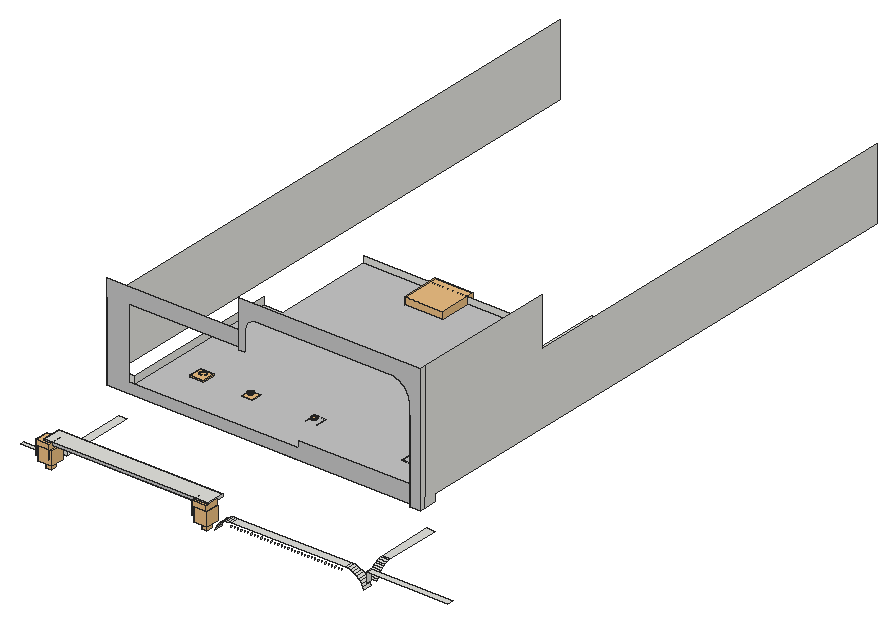
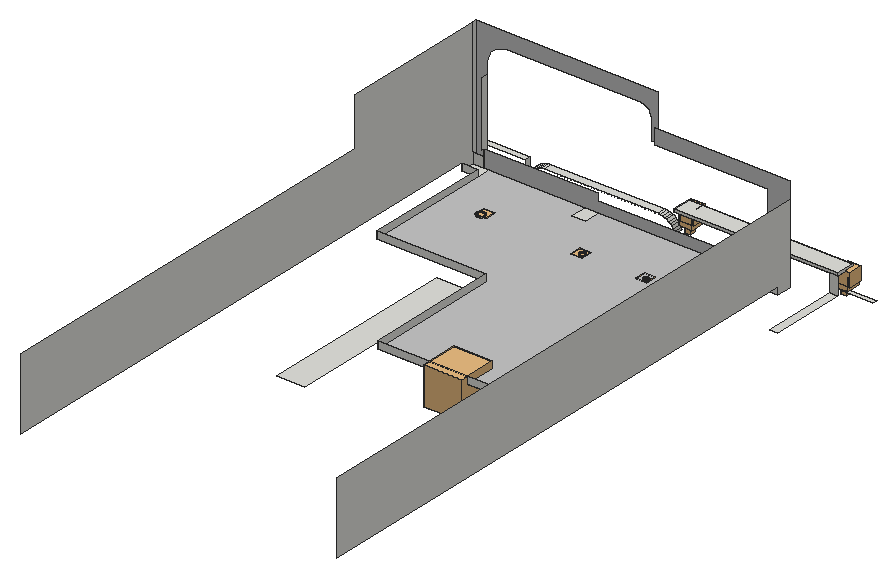
# SketchUp Ruby script. Lengths in inches.
U = 1.inch
M = Sketchup.active_model
def pt(a) = Geom::Point3d.new(a.map { |v| v * U })
def face(e, loops, mat)
  f = e.add_face(loops[0].map { |a| pt(a) })
  loops[1..].each { |l| e.add_face(l.map { |a| pt(a) }).erase! }
  f.material = f.back_material = mat if mat
  f
end
# faces: each face lists its corners as indices into pts; further lists are holes
def faces(e, pts, list, mat = nil) = list.each { |f| face(e, (f[0].is_a?(Array) ? f : [f]).map { |l| l.map { |i| pts[i] } }, mat) }
# xy, xz, yz: faces in a plane at the given z, y or x. An outline is a flat list of corners, or four numbers for a rectangle; further outlines are holes
def ring(l) = l.size == 4 ? [[l[0], l[1]], [l[2], l[1]], [l[2], l[3]], [l[0], l[3]]] : l.each_slice(2).to_a
def flat(e, list, mat, &to3) = list.each { |f| face(e, (f[0].is_a?(Array) ? f : [f]).map { |l| ring(l).map { |u, v| to3.(u, v) } }, mat) }
def xy(e, z, list, mat = nil) = flat(e, list, mat) { |x, y| [x, y, z] }
def xz(e, y, list, mat = nil) = flat(e, list, mat) { |x, z| [x, y, z] }
def yz(e, x, list, mat = nil) = flat(e, list, mat) { |y, z| [x, y, z] }
def lines(e, pts, list) = list.each { |a, b| e.add_line(pt(pts[a]), pt(pts[b])) }
# prism: a flat outline (further loops are holes) pulled along v
def prism(e, loops, v, mat = nil)
  f = face(e, loops, mat); d = Geom::Vector3d.new(v.map { |x| x * U })
  f.pushpull(f.normal.samedirection?(d) ? d.length : -d.length)
end
def box(e, o, s, mat = nil) = prism(e, [[o, [o[0] + s[0], o[1], o[2]], [o[0] + s[0], o[1] + s[1], o[2]], [o[0], o[1] + s[1], o[2]]]], [0, 0, s[2]], mat)
def at(x, y, z, deg = 0) = Geom::Transformation.translation(pt([x, y, z])) * Geom::Transformation.rotation(ORIGIN, Z_AXIS, deg.degrees)
def axes(o, x, y, z) = Geom::Transformation.new([*x, 0, *y, 0, *z, 0, *pt(o).to_a, 1])
def part(name) = M.definitions.add(name)
# library, detail: a bought-in or finely detailed component or shape, given as its bounding box
def library(name, o, s) = part(name).tap { |d| box(d.entities, o, s) }
def detail(e, o, s) = box(e.add_group.entities, o, s)
def put(e, d, t, mat = nil) = e.add_instance(d, t).tap { |i| i.material = mat if mat }
def group(e, t, mat = nil) = e.add_group.tap { |g| g.transformation = t; g.material = mat if mat }.entities
root = M.entities
M.materials.add("[Color M02]").color = [198, 198, 198]
M.materials.add("[Wood Floor Parquet]").color = [145, 89, 39]
c1 = library("Spot Light\#6",[-5.1,-5.1,-11.05],[10.2,10.2,11.05])
c2 = library("Omni Light\#11",[-12,-12,-12],[24,24,24])
c3 = library("Omni Light\#12",[-12,-12,-12],[24,24,24])
c4 = library("Omni Light\#13",[-12,-12,-12],[24,24,24])
c5 = library("Omni Light\#19",[-12,-12,-12],[24,24,24])
c6 = library("Omni Light\#18",[-12,-12,-12],[24,24,24])
c7 = library("Omni Light\#23",[-12,-12,-12],[24,24,24])
c8 = library("Omni Light\#20",[-12,-12,-12],[24,24,24])
c9 = library("Omni Light\#16",[-12,-12,-12],[24,24,24])
c10 = library("Omni Light\#17",[-12,-12,-12],[24,24,24])
c11 = library("Omni Light\#22",[-12,-12,-12],[24,24,24])
c12 = library("Omni Light\#15",[-12,-12,-12],[24,24,24])
c13 = library("Omni Light\#21",[-12,-12,-12],[24,24,24])
c14 = library("Omni Light\#14",[-12,-12,-12],[24,24,24])
c15 = library("Spot Light\#10",[-5.1,-5.1,-11.05],[10.2,10.2,11.05])
xy(root,48,[[52.9375,113,66.86,244.9375]])
xy(root,49.42,[[56.17,85.5625,62.99,89.5625],[330.61,85.5625,337.42,89.5625]],"[Color M02]")
xy(root,50.9375,[[0,94.125,52.9375,101.45]])
xy(root,61.1875,[[376.11,89.5625,576.66,104.0625],[596.33,146.41,610.25,244.9375]])
xy(root,61.98,[[56.17,85.5625,62.99,89.5625],[330.61,85.5625,337.42,89.5625]],"[Color M02]")
xy(root,63.75,[[610.25,94.125,754.3125,104.0625]])
xy(root,79.6875,[[52.9375,79.3125,66.86,89.5625],[66.86,79.3125,66.86,113,341.76,113,341.76,104.75,326.57,104.75,326.57,79.3125],[326.57,79.3125,341.76,89.5625],[52.9375,89.5625,66.86,113],[326.57,89.5625,341.76,104.75]])
xy(root,84,[[52.9375,79.3125,341.76,113],[427.3,467.53,475.3,820.03],[115.1,706.78,146.03,752.85],[181,706.78,229,752.85]])
xy(root,107.6875,[[591.56,213,610.25,219.25],[52.9375,219.25,80.78,244.9375],[388.4375,219.25,412.5,248.6],[582.4,219.25,610.25,244.9375]])
xy(root,107.6875,[[[80.78,219.25,80.78,529.39,115.1,529.39,115.1,706.78,388.8,706.78,388.8,467.53,582.4,467.53,582.4,219.25,412.5,219.25,412.5,248.6,388.4375,248.6,388.4375,219.25],[512.63,317.48,514.56,317.74,516.35,318.48,517.89,319.66,519.07,321.2,519.82,323,520.07,324.92,519.82,326.85,519.07,328.64,517.89,330.18,516.35,331.36,514.56,332.1,512.63,332.36,510.71,332.1,508.91,331.36,507.375,330.18,506.19,328.64,505.45,326.85,505.2,324.92,505.45,323,506.19,321.2,507.375,319.66,508.91,318.48,510.71,317.74],[333.76,319.66,335.12,319.84,336.39,320.37,337.48,321.2,338.3125,322.29,338.84,323.56,339.02,324.92,338.84,326.28,338.3125,327.55,337.48,328.64,336.39,329.47,335.12,330,333.76,330.18,332.4,330,331.13,329.47,330.04,328.64,329.21,327.55,328.68,326.28,328.5,324.92,328.68,323.56,329.21,322.29,330.04,321.2,331.13,320.37,332.4,319.84],[137.46,319.67,138.82,319.85,140.09,320.375,141.17,321.21,142.01,322.3,142.53,323.5625,142.71,324.92,142.53,326.28,142.01,327.55,141.17,328.63,140.09,329.47,138.82,329.99,137.46,330.17,136.1,329.99,134.84,329.47,133.75,328.63,132.91,327.55,132.39,326.28,132.21,324.92,132.39,323.5625,132.91,322.3,133.75,321.21,134.84,320.375,136.1,319.85],[221.33,320.11,222.57,320.27,223.73,320.75,224.73,321.52,225.5,322.51,225.98,323.67,226.14,324.92,225.98,326.17,225.5,327.33,224.73,328.32,223.73,329.09,222.57,329.57,221.33,329.73,220.08,329.57,218.92,329.09,217.92,328.32,217.16,327.33,216.68,326.17,216.51,324.92,216.68,323.67,217.16,322.51,217.92,321.52,218.92,320.75,220.08,320.27]]],"[Color M02]")
xz(root,79.3125,[[52.9375,79.6875,341.76,84]],"[Color M02]")
xz(root,85.5625,[[56.17,49.42,62.99,61.98],[330.61,49.42,337.42,61.98]],"[Wood Floor Parquet]")
xz(root,113,[[52.9375,48,66.86,79.6875],[52.9375,79.6875,341.76,84]])
xz(root,213,[[591.56,107.6875,610.25,107.6875,610.25,331.6875,290.41,331.6875,290.41,249.875,300.96,249.875,300.96,283.625,301.125,286.24,301.61,288.8125,302.41,291.31,303.52,293.68,304.91,295.9,306.5625,297.93,308.46,299.74,310.5625,301.3,312.84,302.58,315.27,303.58,317.79,304.26,320.39,304.625,554.68,304.625,559.5,304.31,564.23,303.37,568.79,301.82,573.12,299.6875,577.13,297.01,580.76,293.83,583.9375,290.2,586.62,286.19,588.75,281.87,590.3,277.3,591.24,272.57,591.56,267.76]],"[Color M02]")
xz(root,219.25,[[591.56,107.6875,610.25,126]])
xz(root,219.25,[[52.9375,107.6875,591.56,107.6875,591.56,138.5625,390.47,138.5625,390.47,126.375,91.81,126.375,91.81,246,91.94,246,91.94,249.875,290.41,249.875,290.41,277.0625,52.9375,277.0625]],"[Color M02]")
xz(root,244.9375,[[52.9375,107.6875,80.78,120],[582.4,107.6875,610.25,120]])
xz(root,467.53,[[388.8,107.6875,582.4,120]])
xz(root,706.78,[[115.1,107.6875,388.8,120]])
yz(root,52.9375,[[79.3125,79.6875,113,84],[219.25,107.6875,219.25,246,1217.1875,246,1217.1875,120,244.9375,120,244.9375,107.6875]])
yz(root,56.17,[[85.5625,49.42,89.5625,61.98]],"[Color M02]")
yz(root,62.99,[[85.5625,49.42,89.5625,61.98]],"[Wood Floor Parquet]")
yz(root,80.78,[[244.9375,107.6875,529.39,120]])
yz(root,330.61,[[85.5625,49.42,89.5625,61.98]],"[Color M02]")
yz(root,337.42,[[85.5625,49.42,89.5625,61.98]],"[Color M02]")
yz(root,341.76,[[79.3125,79.6875,113,84]])
yz(root,373.05,[[92.0625,52.27,92.8125,53.85]])
yz(root,378.96,[[92.0625,52.27,92.8125,54.05]])
yz(root,384.88,[[92.0625,52.27,92.8125,54.05]])
yz(root,388.8,[[467.53,107.6875,706.78,120]])
yz(root,390.79,[[92.0625,52.27,92.8125,54.05]])
yz(root,396.71,[[92.0625,52.27,92.8125,54.05]])
yz(root,402.625,[[92.0625,52.27,92.8125,54.05]])
yz(root,408.54,[[92.0625,52.27,92.8125,54.05]])
yz(root,414.45,[[92.0625,52.27,92.8125,54.05]])
yz(root,420.37,[[92.0625,52.27,92.8125,54.05]])
yz(root,426.28,[[92.0625,52.27,92.8125,54.05]])
yz(root,432.2,[[92.0625,52.27,92.8125,54.05]])
yz(root,438.11,[[92.0625,52.27,92.8125,54.05]])
yz(root,444.03,[[92.0625,52.27,92.8125,54.05]])
yz(root,449.94,[[92.0625,52.27,92.8125,54.05]])
yz(root,455.86,[[92.0625,52.27,92.8125,54.05]])
yz(root,461.77,[[92.0625,52.27,92.8125,54.05]])
yz(root,467.6875,[[92.0625,52.27,92.8125,54.05]])
yz(root,473.6,[[92.0625,52.27,92.8125,54.05]])
yz(root,479.52,[[92.0625,52.27,92.8125,54.05]])
yz(root,485.43,[[92.0625,52.27,92.8125,54.05]])
yz(root,491.35,[[92.0625,52.27,92.8125,54.05]])
yz(root,497.26,[[92.0625,52.27,92.8125,54.05]])
yz(root,503.18,[[92.0625,52.27,92.8125,54.05]])
yz(root,509.09,[[92.0625,52.27,92.8125,54.05]])
yz(root,515,[[92.0625,52.27,92.8125,54.05]])
yz(root,520.92,[[92.0625,52.27,92.8125,54.05]])
yz(root,526.83,[[92.0625,52.27,92.8125,54.05]])
yz(root,532.75,[[92.0625,52.27,92.8125,54.05]])
yz(root,538.66,[[92.0625,52.27,92.8125,54.05]])
yz(root,544.58,[[92.0625,52.27,92.8125,54.05]])
yz(root,550.49,[[92.0625,50.58,92.8125,52.27],[92.0625,52.27,92.8125,54.05]])
yz(root,556.41,[[92.0625,52.27,92.8125,54.05]])
yz(root,562.32,[[92.0625,52.27,92.8125,54.05]])
yz(root,568.24,[[92.0625,52.27,92.8125,54.05]])
yz(root,582.4,[[244.9375,107.6875,467.53,120]])
yz(root,591.56,[[213,107.6875,213,251.38,222.9375,251.38,222.9375,138.5625,219.25,138.5625,219.25,107.6875]])
yz(root,610.25,[[94.125,45.67,104.0625,63.75],[213,107.6875,219.25,107.6875,219.25,126,222.9375,126,222.9375,331.6875,213,331.6875],[219.25,107.6875,244.9375,107.6875,244.9375,120,1217.1875,120,1217.1875,246,479.76,246,479.76,331.6875,222.9375,331.6875,222.9375,126,219.25,126]])
p = [[607.69,104.0625,40.45],[607.69,89.5625,40.45],[609.11,89.5625,36.29],[609.11,104.0625,36.29],[346.56,104.0625,38.51],[346.56,89.5625,38.51],
  [347.85,89.5625,42.3],[347.85,104.0625,42.3],[610.25,116.85,38.51],[610.25,118.14,42.3],[596.33,118.14,42.3],[596.33,116.85,38.51],
  [605.75,104.0625,44.39],[605.75,89.5625,44.39],[349.62,89.5625,45.89],[349.62,104.0625,45.89],[610.25,119.91,45.89],[596.33,119.91,45.89],
  [603.31,104.0625,48.04],[603.31,89.5625,48.04],[351.84,89.5625,49.22],[351.84,104.0625,49.22],[610.25,122.13,49.22],[596.33,122.13,49.22],
  [600.41,104.0625,51.35],[600.41,89.5625,51.35],[354.48,89.5625,52.23],[354.48,104.0625,52.23],[610.25,124.77,52.23],[596.33,124.77,52.23],
  [597.11,104.0625,54.25],[597.11,89.5625,54.25],[357.49,89.5625,54.87],[357.49,104.0625,54.87],[610.25,127.78,54.87],[596.33,127.78,54.87],
  [593.45,104.0625,56.6875],[593.45,89.5625,56.6875],[360.8125,89.5625,57.09],[360.8125,104.0625,57.09],[610.25,131.11,57.09],[596.33,131.11,57.09],
  [589.51,104.0625,58.63],[589.51,89.5625,58.63],[364.4,89.5625,58.86],[364.4,104.0625,58.86],[610.25,134.7,58.86],[596.33,134.7,58.86],
  [585.35,104.0625,60.04],[585.35,89.5625,60.04],[368.19,89.5625,60.15],[368.19,104.0625,60.15],[610.25,138.49,60.15],[596.33,138.49,60.15],
  [581.04,104.0625,60.9],[581.04,89.5625,60.9],[372.12,89.5625,60.93],[372.12,104.0625,60.93],[610.25,142.41,60.93],[596.33,142.41,60.93],
  [376.11,89.5625,61.1875],[376.11,104.0625,61.1875],[576.66,104.0625,61.1875],[576.66,89.5625,61.1875],[610.25,146.41,61.1875],[596.33,146.41,61.1875],
  [512.63,317.48,107.6875],[510.71,317.74,107.6875],[510.71,317.74,109.25],[512.63,317.48,109.25],[514.56,317.74,107.6875],[514.56,317.74,109.25],
  [508.91,318.48,107.6875],[508.91,318.48,109.25],[516.35,318.48,107.6875],[516.35,318.48,109.25],[507.375,319.66,107.6875],[507.375,319.66,109.25],
  [517.89,319.66,107.6875],[517.89,319.66,109.25],[137.46,319.67,107.6875],[136.1,319.85,107.6875],[136.1,319.85,109.25],[137.46,319.67,109.25],
  [138.82,319.85,107.6875],[138.82,319.85,109.25],[333.76,319.66,107.6875],[332.4,319.84,107.6875],[332.4,319.84,109.25],[333.76,319.66,109.25],
  [335.12,319.84,107.6875],[335.12,319.84,109.25],[506.19,321.2,107.6875],[506.19,321.2,109.25],[519.07,321.2,107.6875],[519.07,321.2,109.25],
  [134.84,320.375,107.6875],[134.84,320.375,109.25],[140.09,320.375,107.6875],[140.09,320.375,109.25],[331.13,320.37,107.6875],[331.13,320.37,109.25],
  [336.39,320.37,107.6875],[336.39,320.37,109.25],[221.33,320.11,107.6875],[220.08,320.27,107.6875],[220.08,320.27,109.25],[221.33,320.11,109.25],
  [222.57,320.27,107.6875],[222.57,320.27,109.25],[218.92,320.75,107.6875],[218.92,320.75,109.25],[223.73,320.75,107.6875],[223.73,320.75,109.25],
  [133.75,321.21,107.6875],[133.75,321.21,109.25],[141.17,321.21,107.6875],[141.17,321.21,109.25],[330.04,321.2,107.6875],[330.04,321.2,109.25],
  [337.48,321.2,107.6875],[337.48,321.2,109.25],[217.92,321.52,107.6875],[217.92,321.52,109.25],[224.73,321.52,107.6875],[224.73,321.52,109.25],
  [132.91,322.3,107.6875],[132.91,322.3,109.25],[142.01,322.3,107.6875],[142.01,322.3,109.25],[329.21,322.29,107.6875],[329.21,322.29,109.25],
  [338.3125,322.29,107.6875],[338.3125,322.29,109.25],[505.45,323,107.6875],[505.45,323,109.25],[519.82,323,107.6875],[519.82,323,109.25],
  [217.16,322.51,107.6875],[217.16,322.51,109.25],[225.5,322.51,107.6875],[225.5,322.51,109.25],[132.39,323.5625,107.6875],[132.39,323.5625,109.25],
  [142.53,323.5625,107.6875],[142.53,323.5625,109.25],[328.68,323.56,107.6875],[328.68,323.56,109.25],[338.84,323.56,107.6875],[338.84,323.56,109.25],
  [216.68,323.67,107.6875],[216.68,323.67,109.25],[225.98,323.67,107.6875],[225.98,323.67,109.25],[505.2,324.92,107.6875],[505.2,324.92,109.25],
  [520.07,324.92,107.6875],[520.07,324.92,109.25],[132.21,324.92,107.6875],[132.21,324.92,109.25],[142.71,324.92,107.6875],[142.71,324.92,109.25],
  [328.5,324.92,107.6875],[328.5,324.92,109.25],[339.02,324.92,107.6875],[339.02,324.92,109.25],[216.51,324.92,107.6875],[216.51,324.92,109.25],
  [226.14,324.92,107.6875],[226.14,324.92,109.25],[132.39,326.28,107.6875],[132.39,326.28,109.25],[142.53,326.28,107.6875],[142.53,326.28,109.25],
  [216.68,326.17,107.6875],[216.68,326.17,109.25],[225.98,326.17,107.6875],[225.98,326.17,109.25],[328.68,326.28,107.6875],[328.68,326.28,109.25],
  [338.84,326.28,107.6875],[338.84,326.28,109.25],[505.45,326.85,107.6875],[505.45,326.85,109.25],[519.82,326.85,107.6875],[519.82,326.85,109.25],
  [217.16,327.33,107.6875],[217.16,327.33,109.25],[225.5,327.33,107.6875],[225.5,327.33,109.25],[132.91,327.55,107.6875],[132.91,327.55,109.25],
  [142.01,327.55,107.6875],[142.01,327.55,109.25],[329.21,327.55,107.6875],[329.21,327.55,109.25],[338.3125,327.55,107.6875],[338.3125,327.55,109.25],
  [506.19,328.64,107.6875],[506.19,328.64,109.25],[519.07,328.64,107.6875],[519.07,328.64,109.25],[217.92,328.32,107.6875],[217.92,328.32,109.25],
  [224.73,328.32,107.6875],[224.73,328.32,109.25],[133.75,328.63,107.6875],[133.75,328.63,109.25],[141.17,328.63,107.6875],[141.17,328.63,109.25],
  [330.04,328.64,107.6875],[330.04,328.64,109.25],[337.48,328.64,107.6875],[337.48,328.64,109.25],[218.92,329.09,107.6875],[218.92,329.09,109.25],
  [223.73,329.09,107.6875],[223.73,329.09,109.25],[134.84,329.47,107.6875],[134.84,329.47,109.25],[140.09,329.47,107.6875],[140.09,329.47,109.25],
  [331.13,329.47,107.6875],[331.13,329.47,109.25],[336.39,329.47,107.6875],[336.39,329.47,109.25],[507.375,330.18,107.6875],[507.375,330.18,109.25],
  [517.89,330.18,107.6875],[517.89,330.18,109.25],[220.08,329.57,107.6875],[220.08,329.57,109.25],[222.57,329.57,107.6875],[222.57,329.57,109.25],
  [136.1,329.99,107.6875],[136.1,329.99,109.25],[138.82,329.99,107.6875],[138.82,329.99,109.25],[332.4,330,107.6875],[332.4,330,109.25],
  [335.12,330,107.6875],[335.12,330,109.25],[221.33,329.73,107.6875],[221.33,329.73,109.25],[137.46,330.17,107.6875],[137.46,330.17,109.25],
  [333.76,330.18,107.6875],[333.76,330.18,109.25],[508.91,331.36,107.6875],[508.91,331.36,109.25],[516.35,331.36,107.6875],[516.35,331.36,109.25],
  [510.71,332.1,107.6875],[510.71,332.1,109.25],[514.56,332.1,107.6875],[514.56,332.1,109.25],[512.63,332.36,107.6875],[512.63,332.36,109.25],
  [388.4375,215.23,107.6875],[388.4375,219.25,107.6875],[581.24,92.0625,53.85],[581.24,92.0625,53.6]]
faces(root,p,[[0,1,2,3],[4,5,6,7],[8,9,10,11],[12,13,1,0],[7,6,14,15],[9,16,17,10],[18,19,13,12],[15,14,20,21],
  [16,22,23,17],[24,25,19,18],[21,20,26,27],[22,28,29,23],[30,31,25,24],[27,26,32,33],[28,34,35,29],[36,37,31,30],
  [33,32,38,39],[34,40,41,35],[42,43,37,36],[39,38,44,45],[40,46,47,41],[48,49,43,42],[45,44,50,51],[46,52,53,47],
  [54,55,49,48],[51,50,56,57],[52,58,59,53],[57,56,60,61],[62,63,55,54],[58,64,65,59],[66,67,68,69],[70,66,69,71],
  [67,72,73,68],[74,70,71,75],[72,76,77,73],[78,74,75,79],[80,81,82,83],[84,80,83,85],[86,87,88,89],[90,86,89,91],
  [76,92,93,77],[94,78,79,95],[81,96,97,82],[98,84,85,99],[87,100,101,88],[102,90,91,103],[104,105,106,107],[108,104,107,109],
  [105,110,111,106],[112,108,109,113],[96,114,115,97],[116,98,99,117],[100,118,119,101],[120,102,103,121],[110,122,123,111],[124,112,113,125],
  [114,126,127,115],[128,116,117,129],[118,130,131,119],[132,120,121,133],[92,134,135,93],[136,94,95,137],[122,138,139,123],[140,124,125,141],
  [126,142,143,127],[144,128,129,145],[130,146,147,131],[148,132,133,149],[138,150,151,139],[152,140,141,153],[134,154,155,135],[156,136,137,157],
  [142,158,159,143],[160,144,145,161],[146,162,163,147],[164,148,149,165],[150,166,167,151],[168,152,153,169],[158,170,171,159],[172,160,161,173],
  [166,174,175,167],[176,168,169,177],[162,178,179,163],[180,164,165,181],[154,182,183,155],[184,156,157,185],[174,186,187,175],[188,176,177,189],
  [170,190,191,171],[192,172,173,193],[178,194,195,179],[196,180,181,197],[182,198,199,183],[200,184,185,201],[186,202,203,187],[204,188,189,205],
  [190,206,207,191],[208,192,193,209],[194,210,211,195],[212,196,197,213],[202,214,215,203],[216,204,205,217],[206,218,219,207],[220,208,209,221],
  [210,222,223,211],[224,212,213,225],[198,226,227,199],[228,200,201,229],[214,230,231,215],[232,216,217,233],[218,234,235,219],[236,220,221,237],
  [222,238,239,223],[240,224,225,241],[230,242,243,231],[242,232,233,243],[234,244,245,235],[244,236,237,245],[238,246,247,239],[246,240,241,247],
  [226,248,249,227],[250,228,229,251],[248,252,253,249],[254,250,251,255],[252,256,257,253],[256,254,255,257]])
lines(root,p,[[258,259],[260,261]])
put(root,c1,at(334.02,87.01,49.41))
put(root,c1,at(59.58,87.01,49.41))
put(root,c2,at(59.58,85.5625,61.98))
put(root,c3,at(334.02,85.5625,61.98))
put(root,c4,axes([264.61,685.78,86.6875],[2.75,0,0],[0,2.75,0],[0,0,2.75]))
put(root,c5,at(54.97,86.1,70.33))
put(root,c6,at(330.35,86.15,71.06))
put(root,c1,axes([59.29,86.37,60.0625],[-1,0,0],[0,1,0],[0,0,-1]))
put(root,c1,axes([59.58,85.5625,60.54],[-0.99886,0,0.04783],[0,1,0],[-0.04783,0,-0.99886]))
put(root,c1,axes([333.31,82.36,61.35],[-0.99886,0,0.04783],[0,1,0],[-0.04783,0,-0.99886]))
put(root,c7,at(511.35,311.63,85.1))
put(root,c8,at(138.1,321.21,85.35))
put(root,c9,at(338.96,316.18,87.02))
put(root,c10,at(511.35,311.63,87.02))
put(root,c11,at(343.63,325.36,87.02))
put(root,c12,at(219.81,328.71,89.82))
put(root,c13,at(231.03,313.27,89.82))
put(root,c14,at(138.1,321.21,97.35))
put(root,c15,axes([141.17,321.21,107.6875],[1.87,0,0],[0,1.87,0],[0,0,1.87]))
put(root,c15,axes([225.42,320.99,107.6875],[1.87,0,0],[0,1.87,0],[0,0,1.87]))
put(root,c15,axes([338.3125,322.29,107.6875],[1.87,0,0],[0,1.87,0],[0,0,1.87]))
put(root,c15,axes([510.71,317.74,107.6875],[1.87,0,0],[0,1.87,0],[0,0,1.87]))
